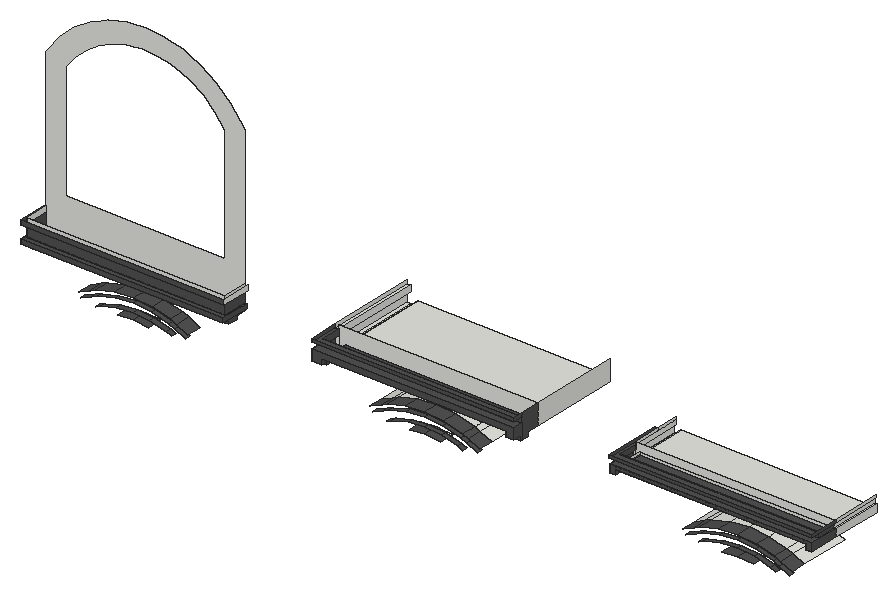
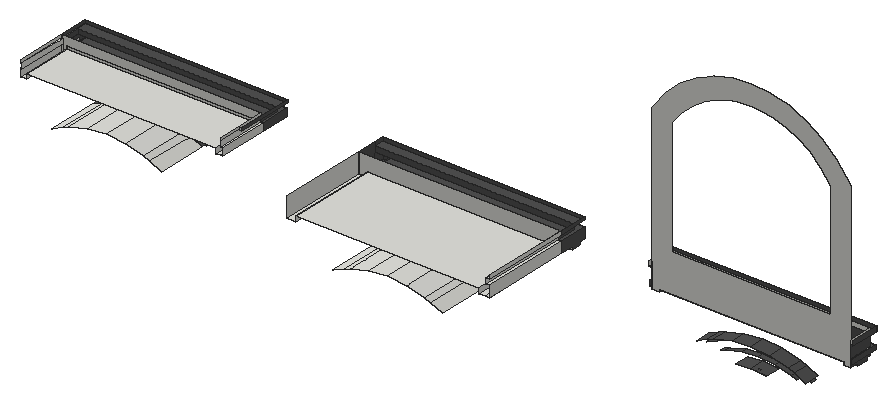
# SketchUp Ruby script. Lengths in inches.
U = 1.inch
M = Sketchup.active_model
def pt(a) = Geom::Point3d.new(a.map { |v| v * U })
def face(e, loops, mat)
  f = e.add_face(loops[0].map { |a| pt(a) })
  loops[1..].each { |l| e.add_face(l.map { |a| pt(a) }).erase! }
  f.material = f.back_material = mat if mat
  f
end
# faces: each face lists its corners as indices into pts; further lists are holes
def faces(e, pts, list, mat = nil) = list.each { |f| face(e, (f[0].is_a?(Array) ? f : [f]).map { |l| l.map { |i| pts[i] } }, mat) }
# xy, xz, yz: faces in a plane at the given z, y or x. An outline is a flat list of corners, or four numbers for a rectangle; further outlines are holes
def ring(l) = l.size == 4 ? [[l[0], l[1]], [l[2], l[1]], [l[2], l[3]], [l[0], l[3]]] : l.each_slice(2).to_a
def flat(e, list, mat, &to3) = list.each { |f| face(e, (f[0].is_a?(Array) ? f : [f]).map { |l| ring(l).map { |u, v| to3.(u, v) } }, mat) }
def xy(e, z, list, mat = nil) = flat(e, list, mat) { |x, y| [x, y, z] }
def xz(e, y, list, mat = nil) = flat(e, list, mat) { |x, z| [x, y, z] }
def yz(e, x, list, mat = nil) = flat(e, list, mat) { |y, z| [x, y, z] }
def lines(e, pts, list) = list.each { |a, b| e.add_line(pt(pts[a]), pt(pts[b])) }
# prism: a flat outline (further loops are holes) pulled along v
def prism(e, loops, v, mat = nil)
  f = face(e, loops, mat); d = Geom::Vector3d.new(v.map { |x| x * U })
  f.pushpull(f.normal.samedirection?(d) ? d.length : -d.length)
end
def box(e, o, s, mat = nil) = prism(e, [[o, [o[0] + s[0], o[1], o[2]], [o[0] + s[0], o[1] + s[1], o[2]], [o[0], o[1] + s[1], o[2]]]], [0, 0, s[2]], mat)
def at(x, y, z, deg = 0) = Geom::Transformation.translation(pt([x, y, z])) * Geom::Transformation.rotation(ORIGIN, Z_AXIS, deg.degrees)
def axes(o, x, y, z) = Geom::Transformation.new([*x, 0, *y, 0, *z, 0, *pt(o).to_a, 1])
def part(name) = M.definitions.add(name)
# library, detail: a bought-in or finely detailed component or shape, given as its bounding box
def library(name, o, s) = part(name).tap { |d| box(d.entities, o, s) }
def detail(e, o, s) = box(e.add_group.entities, o, s)
def put(e, d, t, mat = nil) = e.add_instance(d, t).tap { |i| i.material = mat if mat }
def group(e, t, mat = nil) = e.add_group.tap { |g| g.transformation = t; g.material = mat if mat }.entities
root = M.entities
M.materials.add("[0135_DarkGray]").color = [81, 81, 81]
xy(root,624.16,[[358.47,36.6,363.89,41.66]],"[0135_DarkGray]")
xy(root,624.28,[[64.89,37.34,69.04,44.06]],"[0135_DarkGray]")
xy(root,624.35,[[180.6,37.98,185.57,43.59]],"[0135_DarkGray]")
xy(root,624.78,[[240.7,35.3,246.92,41.28]],"[0135_DarkGray]")
xy(root,625.91,[[64.89,34.6875,69.04,37.34],[64.89,44.06,69.04,49.6875]],"[0135_DarkGray]")
xy(root,626.47,[[180.6,34.6875,185.57,37.98],[180.6,43.59,185.57,49.6875]],"[0135_DarkGray]")
xy(root,626.53,[[240.7,49.6875,242.82,104.375],[242.82,49.6875,246.92,104.375],[358.47,49.6875,363.89,104.375]])
xy(root,626.53,[[240.7,31.6875,246.92,35.3],[358.47,31.6875,363.89,36.6],[240.7,41.28,246.92,49.6875],[358.47,41.66,363.89,49.6875]],"[0135_DarkGray]")
xy(root,627.97,[[69.04,34.6875,180.6,49.6875]],"[0135_DarkGray]")
xy(root,627.98,[[63.89,31.6875,63.89,49.6875,64.89,49.6875,64.89,34.6875,185.57,34.6875,185.57,49.6875,186.64,49.6875,186.64,31.6875]],"[0135_DarkGray]")
xy(root,629.35,[[421.76,49.6875,423.07,80.4375],[423.07,49.6875,425.87,80.4375],[541.16,49.6875,543.95,80.4375],[543.95,49.6875,544.95,80.4375]])
xy(root,629.35,[[421.76,31.6875,425.87,49.6875],[541.16,31.6875,544.95,49.6875]],"[0135_DarkGray]")
xy(root,629.53,[[246.92,49.6875,358.47,104.375]])
xy(root,629.53,[[246.92,31.6875,358.47,49.6875]],"[0135_DarkGray]")
xy(root,630.86,[[63.89,31.6875,186.64,31.6875,186.64,49.6875,185.57,49.6875,185.57,34.6875,64.89,34.6875,64.89,49.6875,63.89,49.6875]],"[0135_DarkGray]")
xy(root,632.35,[[425.87,49.6875,541.16,80.4375]])
xy(root,632.35,[[425.87,31.6875,541.16,49.6875]],"[0135_DarkGray]")
xy(root,633.11,[[240.7,49.6875,242.82,104.375]])
xy(root,633.11,[[240.7,31.6875,363.89,31.6875,363.89,37.6875,242.82,37.6875,242.82,49.6875,240.7,49.6875]],"[0135_DarkGray]")
xy(root,634.06,[[421.76,49.6875,423.07,80.4375],[543.95,49.6875,544.95,80.4375]])
xy(root,634.06,[[421.76,31.6875,544.95,31.6875,544.95,40.6875,543.95,40.6875,543.95,37.6875,423.07,37.6875,423.07,49.6875,421.76,49.6875],[543.95,40.6875,544.95,49.6875]],"[0135_DarkGray]")
xy(root,636.68,[[240.7,49.6875,242.82,104.375]])
xy(root,636.68,[[240.7,31.6875,240.7,49.6875,242.82,49.6875,242.82,37.6875,363.89,37.6875,363.89,31.6875]],"[0135_DarkGray]")
xy(root,637.05,[[543.95,49.6875,544.82,80.4375]])
xy(root,637.05,[[421.14,31.6875,421.14,66.75,423.07,66.75,423.07,37.6875,543.95,37.6875,543.95,31.6875],[543.95,31.6875,544.82,49.6875]],"[0135_DarkGray]")
xy(root,638.17,[[63.64,31.6875,63.64,49.6875,64.89,49.6875,64.89,34.6875,185.57,34.6875,185.57,49.6875,187.39,49.6875,187.39,31.6875]],"[0135_DarkGray]")
xz(root,31.6875,[[425.87,634.06,541.16,634.1]])
xz(root,31.6875,[[240.7,626.53,246.92,626.53,246.92,629.53,358.47,629.53,358.47,626.53,363.89,626.53,363.89,633.11,240.7,633.11],[63.89,627.98,186.64,630.86],[421.76,629.35,425.87,629.35,425.87,632.35,541.16,632.35,541.16,629.35,544.95,629.35,544.95,634.06,421.76,634.06],[240.7,636.68,363.89,638.72],[421.14,637.05,544.82,638.72],
  [63.64,638.17,187.39,641.05]],"[0135_DarkGray]")
xz(root,34.6875,[[64.89,627.98,185.57,630.86],[64.89,638.17,185.57,641.05]])
xz(root,34.6875,[[64.89,625.91,69.04,625.91,69.04,627.97,180.6,627.97,180.6,626.47,185.57,626.47,185.57,627.98,64.89,627.98],[64.89,630.86,185.57,638.17]],"[0135_DarkGray]")
xz(root,35.3,[[240.7,624.78,246.92,626.53]],"[0135_DarkGray]")
xz(root,36.6,[[358.47,624.16,363.89,626.53]],"[0135_DarkGray]")
xz(root,37.34,[[64.89,624.28,69.04,625.91]],"[0135_DarkGray]")
xz(root,37.6875,[[242.82,633.11,363.89,636.68],[423.07,634.06,543.95,637.05]],"[0135_DarkGray]")
xz(root,37.98,[[180.6,624.35,185.57,626.47]],"[0135_DarkGray]")
xz(root,41.28,[[240.7,624.78,246.92,626.53]])
xz(root,41.66,[[358.47,624.16,363.89,626.53]])
xz(root,43.59,[[180.6,624.35,185.57,626.47]])
xz(root,44.06,[[64.89,624.28,69.04,625.91]],"[0135_DarkGray]")
xz(root,49.6875,[[[64.89,625.91,64.89,725.13,73.8125,736.74,82.28,744.61,91.93,750.96,98.9,754.04,102.51,755.63,108.37,757.13,113.71,758.49,125.23,759.45,136.75,758.49,142.09,757.13,147.95,755.63,151.56,754.04,158.52,750.96,168.18,744.61,176.65,736.74,185.57,725.13,185.57,626.47,180.6,626.47,180.6,627.97,69.04,627.97,69.04,625.91],[76.89,650.72,173.57,650.72,173.57,721.05,167.74,728.63,160.74,735.13,152.76,740.39,146.71,743.0625,144.02,744.25,139.12,745.5,134.75,746.61,125.23,747.41,122.29,747.16,116.29,746.66,115.7,746.61,111.33,745.5,106.44,744.25,103.75,743.0625,97.7,740.39,89.72,735.13,82.71,728.63,76.89,721.05]],[240.7,626.53,242.82,633.11],[242.82,626.53,246.92,626.53,246.92,629.53,358.47,629.53,358.47,626.53,363.89,626.53,363.89,638.72,242.82,638.72],[421.76,629.35,423.07,634.06],[423.07,629.35,423.07,638.72,543.95,638.72,543.95,629.35,541.16,629.35,541.16,634.1,425.87,634.1,425.87,629.35],
  [543.95,629.35,544.95,634.06],[425.87,632.35,541.16,634.1]])
xz(root,66.75,[[421.14,637.05,423.07,638.72]])
yz(root,63.64,[[31.6875,638.17,49.6875,641.05]],"[0135_DarkGray]")
yz(root,63.89,[[31.6875,627.98,49.6875,630.86]],"[0135_DarkGray]")
yz(root,64.89,[[34.6875,627.97,34.6875,627.98,49.6875,627.98],[34.6875,627.98,49.6875,630.86],[34.6875,638.17,49.6875,641.05]])
yz(root,64.89,[[37.34,624.28,37.34,625.91,34.6875,625.91,34.6875,627.97,49.6875,627.98,49.6875,625.91,44.06,625.91,44.06,624.28],[34.6875,630.86,49.6875,638.17]],"[0135_DarkGray]")
yz(root,69.04,[[37.34,624.28,44.06,624.28,44.06,625.91,49.6875,625.91,49.6875,627.97,34.6875,627.97,34.6875,625.91,37.34,625.91]])
yz(root,180.6,[[37.98,624.35,37.98,626.47,34.6875,626.47,34.6875,627.97,49.6875,627.97,49.6875,626.47,43.59,626.47,43.59,624.35]],"[0135_DarkGray]")
yz(root,185.57,[[34.6875,627.98,49.6875,630.86],[34.6875,638.17,49.6875,641.05]])
yz(root,185.57,[[37.98,624.35,43.59,624.35,43.59,626.47,49.6875,626.47,49.6875,627.98,34.6875,627.98,34.6875,626.47,37.98,626.47],[34.6875,630.86,49.6875,638.17]],"[0135_DarkGray]")
yz(root,186.64,[[31.6875,627.98,49.6875,630.86]],"[0135_DarkGray]")
yz(root,187.39,[[31.6875,638.17,49.6875,641.05]])
yz(root,240.7,[[49.6875,626.53,104.375,633.11],[49.6875,636.68,104.375,638.72]])
yz(root,240.7,[[35.3,624.78,35.3,626.53,31.6875,626.53,31.6875,633.11,49.6875,633.11,49.6875,626.53,41.28,626.53,41.28,624.78],[31.6875,636.68,49.6875,638.72]],"[0135_DarkGray]")
yz(root,242.82,[[49.6875,633.11,104.375,636.68]])
yz(root,242.82,[[37.6875,633.11,49.6875,636.68]],"[0135_DarkGray]")
yz(root,246.92,[[49.6875,626.53,104.375,629.53]])
yz(root,246.92,[[35.3,624.78,41.28,624.78,41.28,626.53,49.6875,626.53,49.6875,629.53,31.6875,629.53,31.6875,626.53,35.3,626.53]],"[0135_DarkGray]")
yz(root,358.47,[[49.6875,626.53,104.375,629.53]])
yz(root,358.47,[[36.6,624.16,36.6,626.53,31.6875,626.53,31.6875,629.53,49.6875,629.53,49.6875,626.53,41.66,626.53,41.66,624.16]],"[0135_DarkGray]")
yz(root,363.89,[[49.6875,626.53,104.375,638.72]])
yz(root,363.89,[[36.6,624.16,37.6875,624.16,37.6875,633.11,31.6875,633.11,31.6875,626.53,36.6,626.53],[37.6875,624.16,41.66,624.16,41.66,626.53,49.6875,626.53,49.6875,638.72,37.6875,638.72],[31.6875,636.68,37.6875,638.72]],"[0135_DarkGray]")
yz(root,421.14,[[31.6875,637.05,66.75,638.72]],"[0135_DarkGray]")
yz(root,421.76,[[49.6875,629.35,80.4375,634.06]])
yz(root,421.76,[[31.6875,629.35,49.6875,634.06]],"[0135_DarkGray]")
yz(root,423.07,[[49.6875,634.06,80.4375,637.05],[49.6875,637.05,66.75,638.72],[66.75,637.05,80.4375,638.72]])
yz(root,423.07,[[37.6875,634.06,49.6875,637.05]],"[0135_DarkGray]")
yz(root,425.87,[[49.6875,629.35,80.4375,632.35],[40.6875,632.35,49.6875,634.1]])
yz(root,425.87,[[31.6875,629.35,49.6875,632.35]],"[0135_DarkGray]")
yz(root,541.16,[[49.6875,629.35,80.4375,632.35],[40.6875,632.35,49.6875,634.1]])
yz(root,541.16,[[31.6875,629.35,40.6875,632.35],[40.6875,629.35,49.6875,632.35]],"[0135_DarkGray]")
yz(root,543.95,[[49.6875,634.06,80.4375,637.05]])
yz(root,543.95,[[37.6875,634.06,49.6875,637.05]],"[0135_DarkGray]")
yz(root,544.82,[[49.6875,637.05,80.4375,638.72]])
yz(root,544.82,[[31.6875,637.05,49.6875,638.72]],"[0135_DarkGray]")
yz(root,544.95,[[49.6875,629.35,80.4375,634.06]])
yz(root,544.95,[[31.6875,629.35,49.6875,634.06]],"[0135_DarkGray]")
p = [[282.45,43.6875,604.78],[279.47,43.6875,603.46],[279.47,40.6875,603.46],[282.45,40.6875,604.78],[325.49,43.6875,603.46],[322.51,43.6875,604.78],
  [322.51,40.6875,604.78],[325.49,40.6875,603.46],[105.17,43.6875,604.87],[102.18,43.6875,603.55],[102.18,40.6875,603.55],[105.17,40.6875,604.87],
  [115.7,49.6875,603.55],[122.29,49.6875,604.1],[125.23,49.6875,604.35],[125.23,40.6875,604.35],[115.7,40.6875,603.55],[134.75,49.6875,603.55],
  [134.75,40.6875,603.55],[148.28,43.6875,603.55],[145.29,43.6875,604.87],[145.29,40.6875,604.87],[148.28,40.6875,603.55],[292.95,49.6875,603.55],
  [302.48,49.6875,604.35],[302.48,40.6875,604.35],[292.95,40.6875,603.55],[305.64,49.6875,604.08],[305.64,47.6875,604.08],[311.64,47.6875,603.58],
  [311.64,49.6875,603.58],[312,49.6875,603.55],[312,40.6875,603.55],[482.95,49.6875,603.55],[483.7,49.6875,603.61],[483.7,47.6875,603.61],
  [489.7,47.6875,604.11],[489.7,49.6875,604.11],[492.48,49.6875,604.35],[492.48,40.6875,604.35],[482.95,40.6875,603.55],[502,49.6875,603.55],
  [502,40.6875,603.55],[116.29,49.6875,603.55],[116.29,47.6875,603.55],[122.29,47.6875,604.1],[472.16,43.6875,605.64],[469.1,43.6875,604.29],
  [469.1,40.6875,604.29],[472.16,40.6875,605.64],[515.85,43.6875,604.29],[512.8,43.6875,605.64],[512.8,40.6875,605.64],[515.85,40.6875,604.29],
  [292.33,43.6875,607.29],[292.33,40.6875,607.29],[312.63,43.6875,607.29],[312.63,40.6875,607.29],[115.06,43.6875,607.39],[115.06,40.6875,607.39],
  [135.4,43.6875,607.39],[135.4,40.6875,607.39],[460.6875,43.6875,605.14],[467.41,43.6875,608.11],[467.41,40.6875,608.11],[460.6875,40.6875,605.14],
  [517.54,43.6875,608.11],[524.27,43.6875,605.14],[524.27,40.6875,605.14],[517.54,40.6875,608.11],[93.38,43.6875,605.24],[100.12,43.6875,608.22],
  [100.12,40.6875,608.22],[93.38,40.6875,605.24],[150.34,43.6875,608.22],[157.07,43.6875,605.24],[157.07,40.6875,605.24],[150.34,40.6875,608.22],
  [270.53,43.6875,605.4375],[277.28,43.6875,608.42],[277.28,40.6875,608.42],[270.53,40.6875,605.4375],[327.68,43.6875,608.42],[334.43,43.6875,605.4375],
  [334.43,40.6875,605.4375],[327.68,40.6875,608.42],[482.17,43.6875,608.1875],[482.17,40.6875,608.1875],[502.78,43.6875,608.1875],[502.78,40.6875,608.1875],
  [302.48,43.6875,608.14],[302.48,40.6875,608.14],[125.23,43.6875,608.24],[125.23,40.6875,608.24],[98.9,49.6875,610.98],[91.93,49.6875,607.9],
  [91.93,40.6875,607.9],[98.9,40.6875,610.98],[158.52,49.6875,607.9],[151.56,49.6875,610.98],[151.56,40.6875,610.98],[158.52,40.6875,607.9],
  [276.15,49.6875,610.98],[269.18,49.6875,607.9],[269.18,40.6875,607.9],[276.15,40.6875,610.98],[335.77,49.6875,607.9],[328.81,49.6875,610.98],
  [328.81,40.6875,610.98],[335.77,40.6875,607.9],[459.18,49.6875,607.9],[466.15,49.6875,610.98],[466.15,40.6875,610.98],[459.18,40.6875,607.9],
  [518.81,49.6875,610.98],[525.77,49.6875,607.9],[525.77,40.6875,607.9],[518.81,40.6875,610.98],[269.18,104.375,607.9],[276.15,104.375,610.98],
  [328.81,104.375,610.98],[335.77,104.375,607.9],[459.18,80.4375,607.9],[466.15,80.4375,610.98],[518.81,80.4375,610.98],[525.77,80.4375,607.9],
  [470.78,43.6875,609.6],[470.78,40.6875,609.6],[514.17,43.6875,609.6],[514.17,40.6875,609.6],[103.5,43.6875,609.71],[103.5,40.6875,609.71],
  [146.96,43.6875,609.71],[146.96,40.6875,609.71],[492.48,43.6875,609.05],[492.48,40.6875,609.05],[280.68,43.6875,609.92],[280.68,40.6875,609.92],
  [324.28,43.6875,609.92],[324.28,40.6875,609.92],[481.48,43.6875,612.33],[481.48,40.6875,612.33],[503.48,43.6875,612.33],[503.48,40.6875,612.33],
  [114.21,43.6875,612.4375],[114.21,40.6875,612.4375],[136.25,43.6875,612.4375],[136.25,40.6875,612.4375],[291.42,43.6875,612.66],[291.42,40.6875,612.66],
  [313.53,43.6875,612.66],[313.53,40.6875,612.66],[102.51,49.6875,612.57],[102.51,40.6875,612.57],[147.95,49.6875,612.57],[147.95,40.6875,612.57],
  [279.76,49.6875,612.57],[279.76,40.6875,612.57],[325.2,49.6875,612.57],[325.2,40.6875,612.57],[469.76,49.6875,612.57],[469.76,40.6875,612.57],
  [515.2,49.6875,612.57],[515.2,40.6875,612.57],[279.76,104.375,612.57],[325.2,104.375,612.57],[469.76,80.4375,612.57],[515.2,80.4375,612.57],
  [492.48,43.6875,613.25],[492.48,40.6875,613.25],[125.23,43.6875,613.36],[125.23,40.6875,613.36],[113.71,49.6875,615.43],[113.71,40.6875,615.43],
  [136.75,49.6875,615.43],[136.75,40.6875,615.43],[290.96,49.6875,615.43],[290.96,40.6875,615.43],[314,49.6875,615.43],[314,40.6875,615.43],
  [480.96,49.6875,615.43],[480.96,40.6875,615.43],[504,49.6875,615.43],[504,40.6875,615.43],[290.96,104.375,615.43],[314,104.375,615.43],
  [480.96,80.4375,615.43],[504,80.4375,615.43],[302.48,43.6875,613.58],[302.48,40.6875,613.58],[125.23,49.6875,616.39],[125.23,40.6875,616.39],
  [302.48,49.6875,616.39],[302.48,40.6875,616.39],[492.48,49.6875,616.39],[492.48,40.6875,616.39],[302.48,104.375,616.39],[492.48,80.4375,616.39],
  [64.89,49.6875,627.98],[68.99,49.6875,627.98],[242.82,37.6875,629.53],[242.82,37.6875,633.11],[242.82,37.6875,636.68],[242.82,37.6875,638.72],
  [543.95,37.6875,634.06],[543.95,37.6875,632.35],[541.16,40.6875,634.1],[541.16,31.6875,634.1]]
faces(root,p,[[0,1,2,3],[4,5,6,7],[8,9,10,11],[12,13,14,15,16],[14,17,18,15],[19,20,21,22],[23,24,25,26],[24,27,28,29,30,31,32,25],
  [33,34,35,36,37,38,39,40],[38,41,42,39],[46,47,48,49],[50,51,52,53],[54,0,3,55],[5,56,57,6],[58,8,11,59],[20,60,61,21],
  [62,63,64,65],[66,67,68,69],[70,71,72,73],[74,75,76,77],[78,79,80,81],[82,83,84,85],[86,46,49,87],[51,88,89,52],
  [90,54,55,91],[56,90,91,57],[92,58,59,93],[60,92,93,61],[94,95,96,97],[98,99,100,101],[102,103,104,105],[106,107,108,109],
  [110,111,112,113],[114,115,116,117],[63,126,127,64],[128,66,69,129],[71,130,131,72],[132,74,77,133],[134,86,87,135],[88,134,135,89],
  [79,136,137,80],[138,82,85,139],[126,140,141,127],[142,128,129,143],[130,144,145,131],[146,132,133,147],[136,148,149,137],[150,138,139,151],
  [152,94,97,153],[99,154,155,100],[156,102,105,157],[107,158,159,108],[111,160,161,112],[162,114,117,163],[140,168,169,141],[168,142,143,169],
  [144,170,171,145],[170,146,147,171],[172,152,153,173],[154,174,175,155],[176,156,157,177],[158,178,179,159],[160,180,181,161],[182,162,163,183],
  [148,188,189,149],[188,150,151,189],[190,172,173,191],[174,190,191,175],[192,176,177,193],[178,192,193,179],[180,194,195,181],[194,182,183,195]],"[0135_DarkGray]")
faces(root,p,[[13,43,44,45],[27,30,29,28],[34,37,36,35],[102,103,118,119],[106,107,120,121],[111,110,122,123],[115,114,124,125],[156,102,119,164],
  [107,158,165,120],[160,111,123,166],[114,162,167,124],[176,156,164,184],[158,178,185,165],[180,160,166,186],[162,182,187,167],[192,176,184,196],
  [178,192,196,185],[194,180,186,197],[182,194,197,187]])
lines(root,p,[[198,199],[200,201],[202,203],[204,205],[206,207]])
